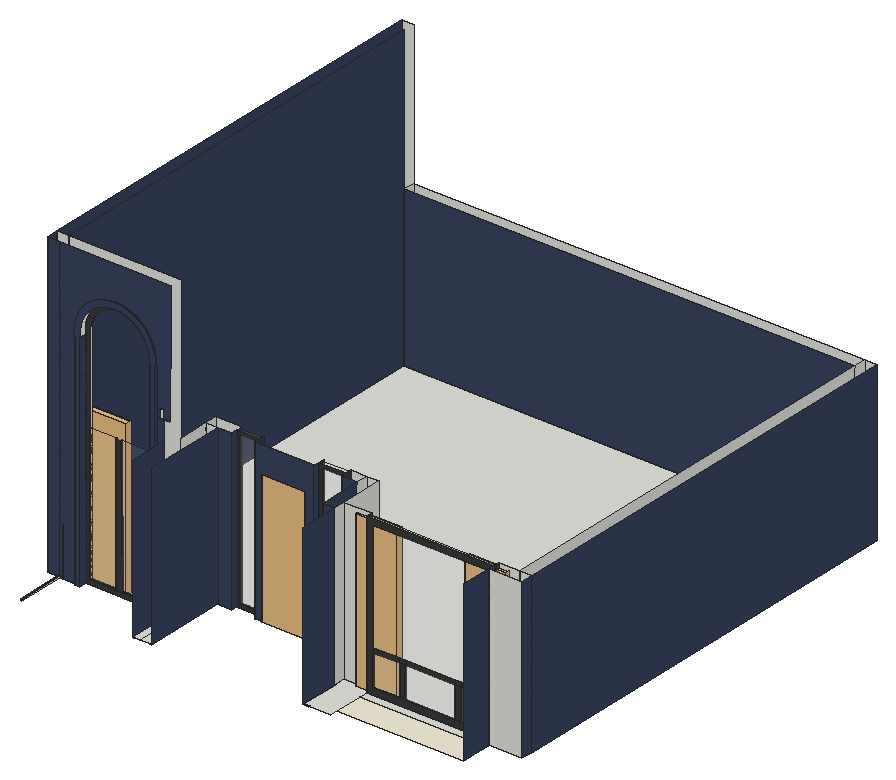
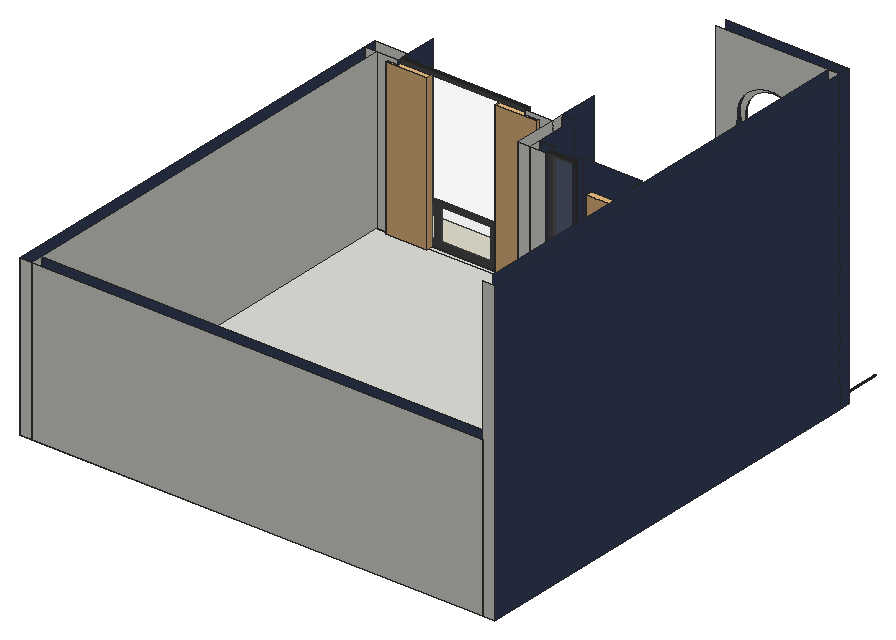
# SketchUp Ruby script. Lengths in inches.
U = 1.inch
M = Sketchup.active_model
def pt(a) = Geom::Point3d.new(a.map { |v| v * U })
def face(e, loops, mat)
  f = e.add_face(loops[0].map { |a| pt(a) })
  loops[1..].each { |l| e.add_face(l.map { |a| pt(a) }).erase! }
  f.material = f.back_material = mat if mat
  f
end
# faces: each face lists its corners as indices into pts; further lists are holes
def faces(e, pts, list, mat = nil) = list.each { |f| face(e, (f[0].is_a?(Array) ? f : [f]).map { |l| l.map { |i| pts[i] } }, mat) }
# xy, xz, yz: faces in a plane at the given z, y or x. An outline is a flat list of corners, or four numbers for a rectangle; further outlines are holes
def ring(l) = l.size == 4 ? [[l[0], l[1]], [l[2], l[1]], [l[2], l[3]], [l[0], l[3]]] : l.each_slice(2).to_a
def flat(e, list, mat, &to3) = list.each { |f| face(e, (f[0].is_a?(Array) ? f : [f]).map { |l| ring(l).map { |u, v| to3.(u, v) } }, mat) }
def xy(e, z, list, mat = nil) = flat(e, list, mat) { |x, y| [x, y, z] }
def xz(e, y, list, mat = nil) = flat(e, list, mat) { |x, z| [x, y, z] }
def yz(e, x, list, mat = nil) = flat(e, list, mat) { |y, z| [x, y, z] }
def lines(e, pts, list) = list.each { |a, b| e.add_line(pt(pts[a]), pt(pts[b])) }
# prism: a flat outline (further loops are holes) pulled along v
def prism(e, loops, v, mat = nil)
  f = face(e, loops, mat); d = Geom::Vector3d.new(v.map { |x| x * U })
  f.pushpull(f.normal.samedirection?(d) ? d.length : -d.length)
end
def box(e, o, s, mat = nil) = prism(e, [[o, [o[0] + s[0], o[1], o[2]], [o[0] + s[0], o[1] + s[1], o[2]], [o[0], o[1] + s[1], o[2]]]], [0, 0, s[2]], mat)
def at(x, y, z, deg = 0) = Geom::Transformation.translation(pt([x, y, z])) * Geom::Transformation.rotation(ORIGIN, Z_AXIS, deg.degrees)
def axes(o, x, y, z) = Geom::Transformation.new([*x, 0, *y, 0, *z, 0, *pt(o).to_a, 1])
def part(name) = M.definitions.add(name)
# library, detail: a bought-in or finely detailed component or shape, given as its bounding box
def library(name, o, s) = part(name).tap { |d| box(d.entities, o, s) }
def detail(e, o, s) = box(e.add_group.entities, o, s)
def put(e, d, t, mat = nil) = e.add_instance(d, t).tap { |i| i.material = mat if mat }
def group(e, t, mat = nil) = e.add_group.tap { |g| g.transformation = t; g.material = mat if mat }.entities
root = M.entities
M.materials.add("0360 AP 9644 Monsoon Midnight-N").color = [56, 67, 95]
M.materials.add("0905 AP 7844 MILD YELLOW").color = [242, 237, 215]
M.materials.add("Glass Clear 001").color = [246, 246, 246]
M.materials["Glass Clear 001"].alpha = 0.1
M.materials.add("[Color M07]").color = [58, 58, 58]
c1 = library("Curtains 004",[-15.59,-2.26,0],[31.18,4.52,116.91])
c2 = library("Door 243 053",[-21.6,-2.79,-0.07],[43.2,5.58,82.64])
xy(root,132,[[112.1875,60.0625,112.1875,89.9375,106.59,89.9375,106.59,88.375,102.41,88.375,102.41,98.79,102.9,98.79,102.9,88.87,106.09,88.87,106.09,90.43,112.68,90.43,112.68,60.55,113.3125,60.55,113.3125,60.0625],[125.0625,60.0625,125.0625,60.55,126.32,60.55,126.32,122.9375,126.8125,122.9375,126.8125,60.0625],[241.5625,60.0625,241.5625,90.43,242.05,90.43,242.05,60.55,246.1875,60.55,246.1875,60.0625],[112.68,60.55,112.68,90.43,106.09,90.43,106.09,88.87,102.9,88.87,102.9,98.79,117.8125,98.79,117.8125,60.55],[117.8125,60.55,126.32,122.9375],
  [242.05,60.55,242.05,90.43,241.5625,90.43,241.5625,98.9375,262.5625,98.9375,262.5625,60.91,262.21,60.91,262.21,60.55],[262.5625,88.27,358.89,94.4375],[45.54,88.375,45.54,89.9375,33.35,89.9375,33.35,90.29,32.51,90.29,32.51,90.43,46.03,90.43,46.03,88.87,49.23,88.87,49.23,98.79,49.72,98.79,49.72,88.375],[46.03,88.87,46.03,90.43,32.51,90.43,32.51,90.29,32.15,90.29,32.15,89.9375,24,89.9375,24,98.79,49.23,98.79,49.23,88.87],[32.15,89.9375,32.51,90.29],
  [32.51,89.9375,33.35,90.29],[232.5625,89.9375,232.5625,123.43,233.05,123.43,233.05,90.43,241.5625,90.43,241.5625,89.9375],[358.89,89.9375,384,98.9375],[233.05,90.43,233.05,123.43,232.5625,123.43,232.5625,131.9375,241.5625,131.9375,241.5625,90.43],[49.72,93.58,102.41,94.96],
  [49.72,94.96,102.41,98.79],[262.5625,96.75,358.89,98.9375],[24,98.79,49.23,98.79,49.23,99.28,102.9,99.28,102.9,98.79,117.8125,98.79,117.8125,131.9375,137.05,131.9375,137.05,132.43,155.05,132.43,155.05,131.9375,199.42,131.9375,199.42,132.43,221.05,132.43,221.05,131.9375,241.5625,131.9375,241.5625,98.9375,375,98.9375,375,416.9375,33,416.9375,33,98.9375,24,98.9375],[49.23,98.79,102.9,99.28],[24,98.9375,33,425.9375],
  [375,98.9375,384,425.9375],[117.8125,122.9375,117.8125,131.9375,137.05,131.9375,137.05,123.43,126.32,123.43,126.32,122.9375],[126.32,122.9375,126.32,123.43,137.05,123.43,137.05,131.9375,137.54,131.9375,137.54,122.9375],[154.56,122.9375,154.56,131.9375,155.05,131.9375,155.05,123.43,160.18,123.43,160.18,122.9375],[192.74,122.9375,192.74,123.43,199.42,123.43,199.42,131.9375,199.92,131.9375,199.92,122.9375],
  [220.5625,122.9375,220.5625,131.9375,221.05,131.9375,221.05,123.43,232.5625,123.43,232.5625,122.9375],[155.05,123.43,199.42,131.9375],[221.05,123.43,232.5625,131.9375],[137.54,130.1875,154.56,131.9375],[199.92,130.1875,220.5625,131.9375],
  [137.05,131.9375,155.05,132.43],[199.42,131.9375,221.05,132.43],[33,416.9375,375,425.9375]])
xy(root,132,[[262.5625,65.9375,358.89,88.27]],"0905 AP 7844 MILD YELLOW")
xy(root,132,[[262.5625,94.4375,358.89,96.75],[137.54,127.4375,154.56,130.1875],[199.92,127.4375,220.5625,130.1875]],"[Color M07]")
xy(root,134.19,[[139.74,127.4375,152.36,128.4375]],"[Color M07]")
xy(root,134.68,[[202.6,127.4375,217.88,128.4375]],"[Color M07]")
xy(root,135.52,[[73.03,93.58,77.87,94.96],[53.24,94.27,73.03,94.96],[77.87,94.27,98.89,94.96]])
xy(root,135.52,[[53.24,93.58,73.03,94.27],[77.87,93.58,98.89,94.27]],"[Color M07]")
xy(root,136.59,[[267.15,94.4375,287.73,95.4375],[291.07,94.4375,329.62,95.4375],[333.85,94.4375,354.31,95.4375]],"[Color M07]")
xy(root,160.8,[[267.15,94.4375,287.73,95.4375],[291.07,94.4375,329.62,95.4375],[333.85,94.4375,354.31,95.4375]],"[Color M07]")
xz(root,88.375,[[45.54,132,49.72,132,49.72,301.29,49.66,302.16,49.63,303.04,49.625,303.91,49.65,304.79,49.71,305.66,49.72,305.77,49.72,301.29,49.66,302.16,49.63,303.04,49.625,303.91,49.65,304.79,49.71,305.66,49.72,305.77,49.79,306.53,49.91,307.4,50.05,308.27,50.22,309.125,50.42,309.98,50.65,310.82,50.9,311.66,51.18,312.49,51.49,313.31,51.83,314.12,52.2,314.91,52.59,315.7,53,316.47,53.44,317.22,53.91,317.96,54.4,318.69,54.91,319.4,55.45,320.09,56.01,320.76,56.59,321.42,57.19,322.05,57.81,322.67,58.46,323.26,59.12,323.84,59.8,324.39,60.5,324.91,61.22,325.42,61.95,325.9,62.7,326.35,63.46,326.78,64.24,327.18,65.03,327.5625,65.83,327.92,66.64,328.24,67.47,328.54,68.3,328.81,69.14,329.05,69.99,329.27,70.84,329.46,71.7,329.61,72.57,329.74,73.44,329.85,74.3125,329.92,75.1875,329.96,76.0625,329.98,76.9375,329.96,77.8125,329.92,78.69,329.85,79.55,329.74,80.42,329.61,81.28,329.46,82.14,329.27,82.99,329.05,83.83,328.81,84.66,328.54,85.48,328.24,86.3,327.92,87.1,327.5625,87.89,327.18,88.66,326.78,89.43,326.35,90.17,325.9,90.91,325.42,91.625,324.91,92.32,324.39,93,323.84,93.67,323.26,94.31,322.67,94.93,322.05,95.54,321.42,96.12,320.76,96.68,320.09,97.21,319.4,97.73,318.69,98.22,317.96,98.68,317.22,99.125,316.47,99.54,315.7,99.93,314.91,100.29,314.12,100.63,313.31,100.94,312.49,101.22,311.66,101.48,310.82,101.71,309.98,101.9,309.125,102.08,308.27,102.22,307.4,102.33,306.53,102.41,305.77,102.42,305.66,102.47,304.79,102.5,303.91,102.5,303.04,102.47,302.16,102.41,301.29,102.41,305.77,102.42,305.66,102.47,304.79,102.5,303.91,102.5,303.04,102.47,302.16,102.41,301.29,102.41,132,106.59,132,106.59,301.15,106.64,301.94,106.63,304.01,106.49,306.08,106.22,308.125,105.8125,310.15,105.28,312.15,104.625,314.11,103.85,316.03,102.95,317.89,101.93,319.69,100.8,321.43,99.56,323.08,98.23,324.66,97.92,324.98,97.2,325.7,96.45,326.38,95.68,327.05,94.89,327.68,94.08,328.29,93.25,328.875,92.41,329.43,91.54,329.96,90.66,330.46,89.76,330.92,88.84,331.36,87.91,331.77,86.97,332.15,86.02,332.49,85.06,332.81,84.08,333.09,83.1,333.34,82.11,333.55,81.11,333.74,80.11,333.89,79.1,334.01,78.09,334.09,77.08,334.14,76.0625,334.16,75.05,334.14,74.04,334.09,73.03,334.01,72.02,333.89,71.02,333.74,70.02,333.55,69.03,333.34,68.04,333.09,67.07,332.81,66.11,332.49,65.15,332.15,64.21,331.77,63.28,331.36,62.37,330.92,61.47,330.46,60.59,329.96,59.72,329.43,58.87,328.875,58.04,328.29,57.23,327.68,56.44,327.05,55.67,326.38,54.93,325.7,54.21,324.98,53.51,324.25,52.84,323.49,52.1875,322.71,51.57,321.91,50.97,321.09,50.4,320.25,49.86,319.39,49.35,318.51,48.87,317.62,48.42,316.71,48,315.79,47.61,314.85,47.25,313.9,46.92,312.94,46.63,311.97,46.36,311,46.13,310.01,45.94,309.01,45.77,308.01,45.64,307.01,45.56,306.17,45.54,306,45.48,304.99,45.44,303.97,45.45,302.96,45.48,301.94,45.54,301.15]],"0360 AP 9644 Monsoon Midnight-N")
xz(root,89.9375,[[32.51,131.3125,33,132],[32.15,132,32.51,132.5625],[32.51,132,33,132,33,132.625,32.59,132.625,32.59,132.5625,32.51,132.5625],[33,132,33.35,132.625],[35.375,132,35.75,168],
  [358.89,132,384,252],[32.15,132.5625,32.51,132.625],[32.51,132.5625,32.59,132.625]])
xz(root,89.9375,[[24,132,32.15,132,32.15,132.8125,33,132.8125,33,360,24,360],[35.75,132,45.54,132,45.54,301.15,45.48,301.94,45.45,302.96,45.44,303.97,45.48,304.99,45.54,306,45.56,306.17,45.64,307.01,45.77,308.01,45.94,309.01,46.13,310.01,46.36,311,46.63,311.97,46.92,312.94,47.25,313.9,47.61,314.85,48,315.79,48.42,316.71,48.87,317.62,49.35,318.51,49.86,319.39,50.4,320.25,50.97,321.09,51.57,321.91,52.1875,322.71,52.84,323.49,53.51,324.25,54.21,324.98,54.93,325.7,55.67,326.38,56.44,327.05,57.23,327.68,58.04,328.29,58.87,328.875,59.72,329.43,60.59,329.96,61.47,330.46,62.37,330.92,63.28,331.36,64.21,331.77,65.15,332.15,66.11,332.49,67.07,332.81,68.04,333.09,69.03,333.34,70.02,333.55,71.02,333.74,72.02,333.89,73.03,334.01,74.04,334.09,75.05,334.14,76.0625,334.16,77.08,334.14,78.09,334.09,79.1,334.01,80.11,333.89,81.11,333.74,82.11,333.55,83.1,333.34,84.08,333.09,85.06,332.81,86.02,332.49,86.97,332.15,87.91,331.77,88.84,331.36,89.76,330.92,90.66,330.46,91.54,329.96,92.41,329.43,93.25,328.875,94.08,328.29,94.89,327.68,95.68,327.05,96.45,326.38,97.2,325.7,97.92,324.98,98.23,324.66,99.56,323.08,100.8,321.43,101.93,319.69,102.95,317.89,103.85,316.03,104.625,314.11,105.28,312.15,105.8125,310.15,106.22,308.125,106.49,306.08,106.63,304.01,106.64,301.94,106.59,301.15,106.59,273.625,112.1875,273.625,112.1875,266.6875,116.8,266.6875,116.8,303.4375,117.8125,303.4375,117.8125,360,33,360,33,132.8125,33.35,132.8125,33.35,132.1875,35.375,132.1875,35.375,168.3125,35.75,168.3125],[33.35,132,35.375,132.1875],[106.59,132,112.1875,266.6875],[232.5625,132,241.5625,252],
  [32.15,132.625,32.51,132.8125],[32.51,132.625,32.59,132.8125],[32.59,132.625,33,132.8125],[33,132.625,33.35,132.8125]],"0360 AP 9644 Monsoon Midnight-N")
xz(root,90.02,[[32.07,132.5625,32.59,132.625]])
xz(root,90.02,[[32.07,132.625,32.59,132.8125]],"0360 AP 9644 Monsoon Midnight-N")
xz(root,93.58,[[[49.72,132,102.41,132,102.41,305.77,102.33,306.53,102.22,307.4,102.08,308.27,101.9,309.125,101.71,309.98,101.48,310.82,101.22,311.66,100.94,312.49,100.63,313.31,100.29,314.12,99.93,314.91,99.54,315.7,99.125,316.47,98.68,317.22,98.22,317.96,97.73,318.69,97.21,319.4,96.68,320.09,96.12,320.76,95.54,321.42,94.93,322.05,94.31,322.67,93.67,323.26,93,323.84,92.32,324.39,91.625,324.91,90.91,325.42,90.17,325.9,89.43,326.35,88.66,326.78,87.89,327.18,87.1,327.5625,86.3,327.92,85.48,328.24,84.66,328.54,83.83,328.81,82.99,329.05,82.14,329.27,81.28,329.46,80.42,329.61,79.55,329.74,78.69,329.85,77.8125,329.92,76.9375,329.96,76.0625,329.98,75.1875,329.96,74.3125,329.92,73.44,329.85,72.57,329.74,71.7,329.61,70.84,329.46,69.99,329.27,69.14,329.05,68.3,328.81,67.47,328.54,66.64,328.24,65.83,327.92,65.03,327.5625,64.24,327.18,63.46,326.78,62.7,326.35,61.95,325.9,61.22,325.42,60.5,324.91,59.8,324.39,59.12,323.84,58.46,323.26,57.81,322.67,57.19,322.05,56.59,321.42,56.01,320.76,55.45,320.09,54.91,319.4,54.4,318.69,53.91,317.96,53.44,317.22,53,316.47,52.59,315.7,52.2,314.91,51.83,314.12,51.49,313.31,51.18,312.49,50.9,311.66,50.65,310.82,50.42,309.98,50.22,309.125,50.05,308.27,49.91,307.4,49.79,306.53,49.72,305.77],[53.24,135.52,53.24,305.6,53.29,306.13,53.39,306.89,53.51,307.64,53.66,308.38,53.83,309.12,54.03,309.85,54.25,310.58,54.49,311.3,54.76,312.01,55.06,312.71,55.37,313.4,55.71,314.08,56.07,314.75,56.45,315.4,56.85,316.05,57.28,316.67,57.72,317.29,58.19,317.89,58.67,318.47,59.18,319.04,59.7,319.59,60.24,320.125,60.8,320.64,61.375,321.13,61.97,321.61,62.57,322.07,63.19,322.51,63.83,322.92,64.48,323.32,65.14,323.6875,65.8125,324.04,66.5,324.37,67.19,324.67,67.9,324.95,68.61,325.21,69.33,325.45,70.06,325.66,70.8,325.85,71.54,326.01,72.28,326.15,73.03,326.26,73.79,326.35,74.55,326.41,75.3,326.45,76.0625,326.46,76.82,326.45,77.58,326.41,78.34,326.35,79.09,326.26,79.84,326.15,80.59,326.01,81.33,325.85,82.06,325.66,82.79,325.45,83.52,325.21,84.23,324.95,84.93,324.67,85.63,324.37,86.3125,324.04,86.99,323.6875,87.65,323.32,88.3,322.92,88.93,322.51,89.55,322.07,90.16,321.61,90.75,321.13,91.32,320.64,91.88,320.125,92.42,319.59,92.95,319.04,93.45,318.47,93.94,317.89,94.4,317.29,94.85,316.67,95.27,316.05,95.67,315.4,96.06,314.75,96.42,314.08,96.75,313.4,97.07,312.71,97.36,312.01,97.63,311.3,97.875,310.58,98.1,309.85,98.29,309.12,98.47,308.38,98.62,307.64,98.74,306.89,98.84,306.13,98.89,305.6,98.89,135.52]],[73.03,135.52,77.87,135.52,76.9,238.39,73.03,238.39]],"[Color M07]")
xz(root,94.27,[[53.24,135.52,73.03,238.39],[77.87,135.52,98.89,135.52,98.89,238.39,76.9,238.39]],"Glass Clear 001")
xz(root,94.4375,[[[262.5625,132,358.89,252],[267.15,136.59,354.31,247.41]],[287.73,136.59,291.07,160.8],[329.62,136.59,333.85,160.8],[267.15,160.8,287.73,164.31],[287.73,160.8,291.07,164.31],
  [291.07,160.8,329.62,164.31],[329.62,160.8,333.85,164.31],[333.85,160.8,354.31,164.31]],"[Color M07]")
xz(root,94.96,[[[49.72,132,49.72,305.77,49.79,306.53,49.91,307.4,50.05,308.27,50.22,309.125,50.42,309.98,50.65,310.82,50.9,311.66,51.18,312.49,51.49,313.31,51.83,314.12,52.2,314.91,52.59,315.7,53,316.47,53.44,317.22,53.91,317.96,54.4,318.69,54.91,319.4,55.45,320.09,56.01,320.76,56.59,321.42,57.19,322.05,57.81,322.67,58.46,323.26,59.12,323.84,59.8,324.39,60.5,324.91,61.22,325.42,61.95,325.9,62.7,326.35,63.46,326.78,64.24,327.18,65.03,327.5625,65.83,327.92,66.64,328.24,67.47,328.54,68.3,328.81,69.14,329.05,69.99,329.27,70.84,329.46,71.7,329.61,72.57,329.74,73.44,329.85,74.3125,329.92,75.1875,329.96,76.0625,329.98,76.9375,329.96,77.8125,329.92,78.69,329.85,79.55,329.74,80.42,329.61,81.28,329.46,82.14,329.27,82.99,329.05,83.83,328.81,84.66,328.54,85.48,328.24,86.3,327.92,87.1,327.5625,87.89,327.18,88.66,326.78,89.43,326.35,90.17,325.9,90.91,325.42,91.625,324.91,92.32,324.39,93,323.84,93.67,323.26,94.31,322.67,94.93,322.05,95.54,321.42,96.12,320.76,96.68,320.09,97.21,319.4,97.73,318.69,98.22,317.96,98.68,317.22,99.125,316.47,99.54,315.7,99.93,314.91,100.29,314.12,100.63,313.31,100.94,312.49,101.22,311.66,101.48,310.82,101.71,309.98,101.9,309.125,102.08,308.27,102.22,307.4,102.33,306.53,102.41,305.77,102.41,132],[53.24,135.52,98.89,135.52,98.89,305.6,98.84,306.13,98.74,306.89,98.62,307.64,98.47,308.38,98.29,309.12,98.1,309.85,97.875,310.58,97.63,311.3,97.36,312.01,97.07,312.71,96.75,313.4,96.42,314.08,96.06,314.75,95.67,315.4,95.27,316.05,94.85,316.67,94.4,317.29,93.94,317.89,93.45,318.47,92.95,319.04,92.42,319.59,91.88,320.125,91.32,320.64,90.75,321.13,90.16,321.61,89.55,322.07,88.93,322.51,88.3,322.92,87.65,323.32,86.99,323.6875,86.3125,324.04,85.63,324.37,84.93,324.67,84.23,324.95,83.52,325.21,82.79,325.45,82.06,325.66,81.33,325.85,80.59,326.01,79.84,326.15,79.09,326.26,78.34,326.35,77.58,326.41,76.82,326.45,76.0625,326.46,75.3,326.45,74.55,326.41,73.79,326.35,73.03,326.26,72.28,326.15,71.54,326.01,70.8,325.85,70.06,325.66,69.33,325.45,68.61,325.21,67.9,324.95,67.19,324.67,66.5,324.37,65.8125,324.04,65.14,323.6875,64.48,323.32,63.83,322.92,63.19,322.51,62.57,322.07,61.97,321.61,61.375,321.13,60.8,320.64,60.24,320.125,59.7,319.59,59.18,319.04,58.67,318.47,58.19,317.89,57.72,317.29,57.28,316.67,56.85,316.05,56.45,315.4,56.07,314.75,55.71,314.08,55.37,313.4,55.06,312.71,54.76,312.01,54.49,311.3,54.25,310.58,54.03,309.85,53.83,309.12,53.66,308.38,53.51,307.64,53.39,306.89,53.29,306.13,53.24,305.6]]])
xz(root,95.4375,[[267.15,136.59,287.73,160.8],[291.07,136.59,329.62,160.8],[333.85,136.59,354.31,160.8]],"Glass Clear 001")
xz(root,96.75,[[262.5625,132,358.89,252]],"Glass Clear 001")
xz(root,98.79,[[24,132,24,360,117.8125,360,117.8125,132,102.41,132,102.41,305.77,102.33,306.53,102.22,307.4,102.08,308.27,101.9,309.125,101.71,309.98,101.48,310.82,101.22,311.66,100.94,312.49,100.63,313.31,100.29,314.12,99.93,314.91,99.54,315.7,99.125,316.47,98.68,317.22,98.22,317.96,97.73,318.69,97.21,319.4,96.68,320.09,96.12,320.76,95.54,321.42,94.93,322.05,94.31,322.67,93.67,323.26,93,323.84,92.32,324.39,91.625,324.91,90.91,325.42,90.17,325.9,89.43,326.35,88.66,326.78,87.89,327.18,87.1,327.5625,86.3,327.92,85.48,328.24,84.66,328.54,83.83,328.81,82.99,329.05,82.14,329.27,81.28,329.46,80.42,329.61,79.55,329.74,78.69,329.85,77.8125,329.92,76.9375,329.96,76.0625,329.98,75.1875,329.96,74.3125,329.92,73.44,329.85,72.57,329.74,71.7,329.61,70.84,329.46,69.99,329.27,69.14,329.05,68.3,328.81,67.47,328.54,66.64,328.24,65.83,327.92,65.03,327.5625,64.24,327.18,63.46,326.78,62.7,326.35,61.95,325.9,61.22,325.42,60.5,324.91,59.8,324.39,59.12,323.84,58.46,323.26,57.81,322.67,57.19,322.05,56.59,321.42,56.01,320.76,55.45,320.09,54.91,319.4,54.4,318.69,53.91,317.96,53.44,317.22,53,316.47,52.59,315.7,52.2,314.91,51.83,314.12,51.49,313.31,51.18,312.49,50.9,311.66,50.65,310.82,50.42,309.98,50.22,309.125,50.05,308.27,49.91,307.4,49.79,306.53,49.72,305.77,49.72,132]])
xz(root,98.9375,[[24,132,33,360],[241.5625,132,262.5625,252],[358.89,132,375,252],[375,132,384,252]])
xz(root,122.9375,[[117.8125,132,126.8125,252]])
xz(root,122.9375,[[126.8125,132,137.54,252],[154.56,132,160.18,132,160.18,231.5,192.74,231.5,192.74,132,199.92,132,199.92,252,154.56,252],[220.5625,132,232.5625,252]],"0360 AP 9644 Monsoon Midnight-N")
xz(root,127.4375,[[[137.54,132,154.56,252],[139.74,134.19,152.36,249.81]],[[199.92,132,220.5625,252],[202.6,134.68,217.88,249.32]]],"[Color M07]")
xz(root,128.4375,[[139.74,134.19,152.36,249.81],[202.6,134.68,217.88,249.32]],"Glass Clear 001")
xz(root,130.1875,[[137.54,132,154.56,252],[199.92,132,220.5625,252]],"Glass Clear 001")
xz(root,131.9375,[[117.8125,132,137.54,252],[220.5625,132,232.5625,252],[232.5625,132,241.5625,252]])
xz(root,416.9375,[[33,132,375,252]],"0360 AP 9644 Monsoon Midnight-N")
xz(root,425.9375,[[24,132,33,360],[33,132,375,252],[375,132,384,252]])
yz(root,24,[[89.9375,132,98.79,360],[98.9375,132,425.9375,360]],"0360 AP 9644 Monsoon Midnight-N")
yz(root,32.07,[[53.9375,132.5625,90.02,132.625],[53.9375,132.625,90.02,132.8125]],"0360 AP 9644 Monsoon Midnight-N")
yz(root,32.15,[[53.9375,132.5625,89.9375,132.625]])
yz(root,32.15,[[53.9375,132.625,89.9375,132.8125]],"0360 AP 9644 Monsoon Midnight-N")
yz(root,32.51,[[53.9375,132,89.9375,132.625]])
yz(root,32.51,[[53.9375,132.625,89.9375,132.8125]],"0360 AP 9644 Monsoon Midnight-N")
yz(root,32.59,[[89.9375,132.5625,90.02,132.625]])
yz(root,32.59,[[53.9375,132.625,89.9375,132.8125],[89.9375,132.625,90.02,132.8125]],"0360 AP 9644 Monsoon Midnight-N")
yz(root,33,[[53.9375,131.3125,89.9375,132.625],[416.9375,132,425.9375,252]])
yz(root,33,[[98.9375,132,416.9375,360],[53.9375,132.625,89.9375,132.8125]],"0360 AP 9644 Monsoon Midnight-N")
yz(root,33.35,[[53.9375,132.625,89.9375,132.8125]],"0360 AP 9644 Monsoon Midnight-N")
yz(root,45.54,[[88.375,132,89.9375,136.18]])
yz(root,45.54,[[88.375,136.18,89.9375,301.15]],"0360 AP 9644 Monsoon Midnight-N")
yz(root,49.72,[[88.375,132,93.58,301.29],[94.96,132,98.79,301.29]],"0360 AP 9644 Monsoon Midnight-N")
yz(root,49.72,[[93.58,132,94.96,301.29]],"[Color M07]")
yz(root,53.24,[[94.27,135.52,94.96,238.39]])
yz(root,53.24,[[93.58,135.52,94.27,238.39]],"[Color M07]")
yz(root,73.03,[[93.58,135.52,94.27,238.39]],"[Color M07]")
yz(root,98.89,[[94.27,135.52,94.96,238.39]])
yz(root,98.89,[[93.58,135.52,94.27,238.39]],"[Color M07]")
yz(root,102.41,[[93.58,132,94.96,301.29]])
yz(root,102.41,[[88.375,132,93.58,301.29],[94.96,132,98.79,301.29]],"0360 AP 9644 Monsoon Midnight-N")
yz(root,106.59,[[88.375,132,89.9375,136.18]])
yz(root,106.59,[[88.375,136.18,89.9375,301.15]],"0360 AP 9644 Monsoon Midnight-N")
yz(root,112.1875,[[60.0625,132,89.9375,252]],"0360 AP 9644 Monsoon Midnight-N")
yz(root,117.8125,[[98.79,132,122.9375,252],[122.9375,132,131.9375,252]])
yz(root,126.8125,[[60.0625,132,122.9375,252]],"0360 AP 9644 Monsoon Midnight-N")
yz(root,137.54,[[122.9375,132,127.4375,252],[130.1875,132,131.9375,252]],"0360 AP 9644 Monsoon Midnight-N")
yz(root,137.54,[[127.4375,132,130.1875,252]],"[Color M07]")
yz(root,139.74,[[127.4375,134.19,128.4375,249.81]],"[Color M07]")
yz(root,152.36,[[127.4375,134.19,128.4375,249.81]],"[Color M07]")
yz(root,154.56,[[122.9375,132,127.4375,252],[130.1875,132,131.9375,252]],"0360 AP 9644 Monsoon Midnight-N")
yz(root,154.56,[[127.4375,132,130.1875,252]],"[Color M07]")
yz(root,160.18,[[122.9375,132,123.43,231.5]],"0360 AP 9644 Monsoon Midnight-N")
yz(root,192.74,[[122.9375,132,123.43,231.5]],"0360 AP 9644 Monsoon Midnight-N")
yz(root,199.92,[[122.9375,132,127.4375,252],[130.1875,132,131.9375,252]],"0360 AP 9644 Monsoon Midnight-N")
yz(root,199.92,[[127.4375,132,130.1875,252]],"[Color M07]")
yz(root,202.6,[[127.4375,134.68,128.4375,249.32]],"[Color M07]")
yz(root,217.88,[[127.4375,134.68,128.4375,249.32]],"[Color M07]")
yz(root,220.5625,[[122.9375,132,127.4375,252],[130.1875,132,131.9375,252]],"0360 AP 9644 Monsoon Midnight-N")
yz(root,220.5625,[[127.4375,132,130.1875,252]],"[Color M07]")
yz(root,232.5625,[[122.9375,132,131.9375,252]])
yz(root,232.5625,[[89.9375,132,122.9375,252]],"0360 AP 9644 Monsoon Midnight-N")
yz(root,241.5625,[[89.9375,132,98.9375,252],[98.9375,132,131.9375,252]])
yz(root,241.5625,[[60.0625,132,89.9375,252]],"0360 AP 9644 Monsoon Midnight-N")
yz(root,262.5625,[[96.75,132,98.9375,252]],"0360 AP 9644 Monsoon Midnight-N")
yz(root,262.5625,[[94.4375,132,96.75,252]],"[Color M07]")
yz(root,267.15,[[94.4375,136.59,95.4375,160.8]],"[Color M07]")
yz(root,287.73,[[94.4375,136.59,95.4375,160.8]],"[Color M07]")
yz(root,291.07,[[94.4375,136.59,95.4375,160.8]],"[Color M07]")
yz(root,329.62,[[94.4375,136.59,95.4375,160.8]],"[Color M07]")
yz(root,333.85,[[94.4375,136.59,95.4375,160.8]],"[Color M07]")
yz(root,354.31,[[94.4375,136.59,95.4375,160.8]],"[Color M07]")
yz(root,358.89,[[65.9375,132,89.9375,252],[89.9375,132,94.4375,252],[96.75,132,98.9375,252]],"0360 AP 9644 Monsoon Midnight-N")
yz(root,358.89,[[94.4375,132,96.75,252]],"[Color M07]")
yz(root,375,[[98.9375,132,416.9375,252],[416.9375,132,425.9375,252]])
yz(root,384,[[89.9375,132,98.9375,252],[98.9375,132,425.9375,252]],"0360 AP 9644 Monsoon Midnight-N")
p = [[77.87,94.27,135.52],[76.9,94.27,238.39],[76.9,93.58,238.39],[77.87,93.58,135.52]]
faces(root,p,[[0,1,2,3]],"[Color M07]")
put(root,c1,at(62.55,98.79,132))
put(root,c1,at(350.85,98.9375,132))
put(root,c1,at(267.81,98.9375,132))
put(root,c2,axes([176.62,125.28,132.08],[-0.76121,0,0],[0,-1,0],[0,0,1.20415]))
